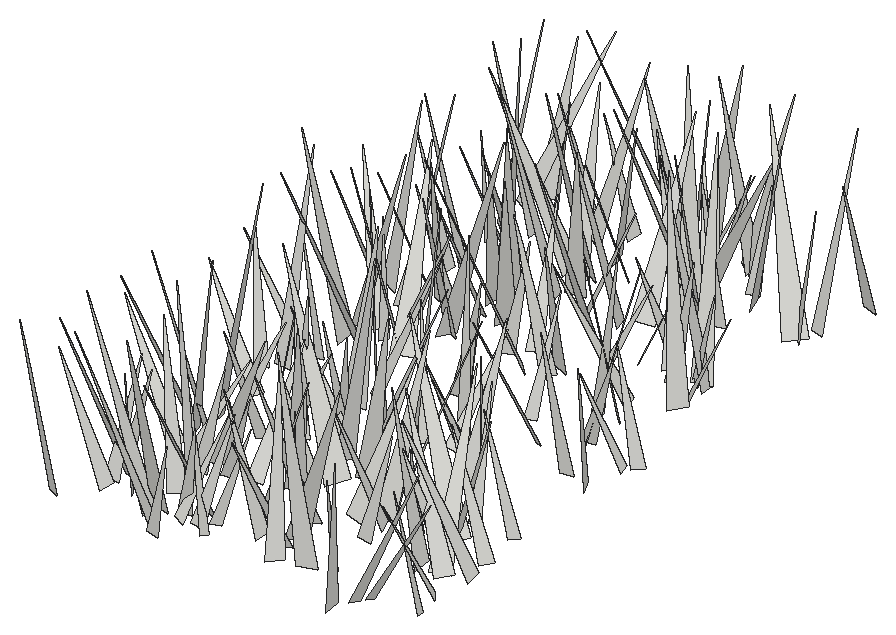
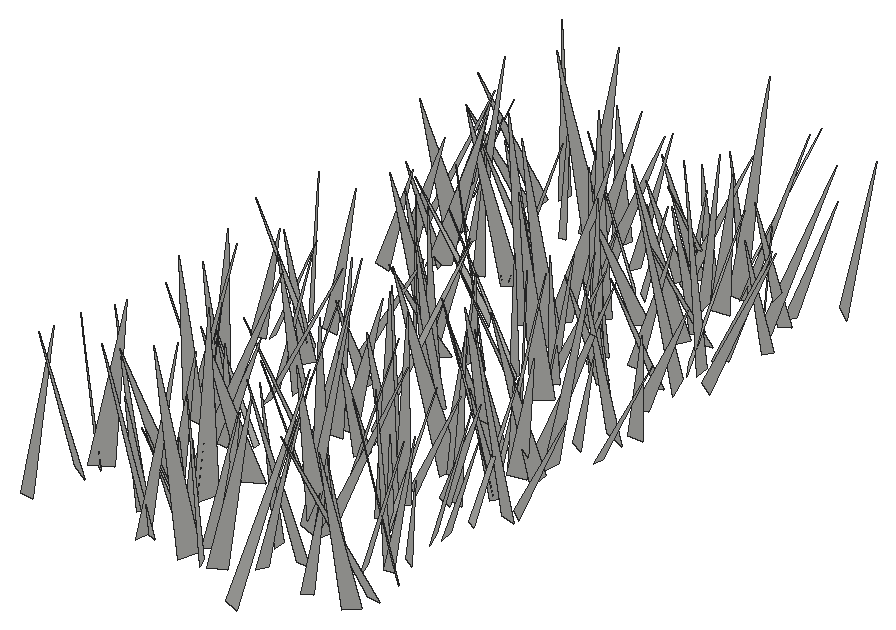
# SketchUp Ruby script. Lengths in inches.
U = 1.inch
M = Sketchup.active_model
def pt(a) = Geom::Point3d.new(a.map { |v| v * U })
def face(e, loops, mat)
  f = e.add_face(loops[0].map { |a| pt(a) })
  loops[1..].each { |l| e.add_face(l.map { |a| pt(a) }).erase! }
  f.material = f.back_material = mat if mat
  f
end
# faces: each face lists its corners as indices into pts; further lists are holes
def faces(e, pts, list, mat = nil) = list.each { |f| face(e, (f[0].is_a?(Array) ? f : [f]).map { |l| l.map { |i| pts[i] } }, mat) }
# xy, xz, yz: faces in a plane at the given z, y or x. An outline is a flat list of corners, or four numbers for a rectangle; further outlines are holes
def ring(l) = l.size == 4 ? [[l[0], l[1]], [l[2], l[1]], [l[2], l[3]], [l[0], l[3]]] : l.each_slice(2).to_a
def flat(e, list, mat, &to3) = list.each { |f| face(e, (f[0].is_a?(Array) ? f : [f]).map { |l| ring(l).map { |u, v| to3.(u, v) } }, mat) }
def xy(e, z, list, mat = nil) = flat(e, list, mat) { |x, y| [x, y, z] }
def xz(e, y, list, mat = nil) = flat(e, list, mat) { |x, z| [x, y, z] }
def yz(e, x, list, mat = nil) = flat(e, list, mat) { |y, z| [x, y, z] }
def lines(e, pts, list) = list.each { |a, b| e.add_line(pt(pts[a]), pt(pts[b])) }
# prism: a flat outline (further loops are holes) pulled along v
def prism(e, loops, v, mat = nil)
  f = face(e, loops, mat); d = Geom::Vector3d.new(v.map { |x| x * U })
  f.pushpull(f.normal.samedirection?(d) ? d.length : -d.length)
end
def box(e, o, s, mat = nil) = prism(e, [[o, [o[0] + s[0], o[1], o[2]], [o[0] + s[0], o[1] + s[1], o[2]], [o[0], o[1] + s[1], o[2]]]], [0, 0, s[2]], mat)
def at(x, y, z, deg = 0) = Geom::Transformation.translation(pt([x, y, z])) * Geom::Transformation.rotation(ORIGIN, Z_AXIS, deg.degrees)
def axes(o, x, y, z) = Geom::Transformation.new([*x, 0, *y, 0, *z, 0, *pt(o).to_a, 1])
def part(name) = M.definitions.add(name)
# library, detail: a bought-in or finely detailed component or shape, given as its bounding box
def library(name, o, s) = part(name).tap { |d| box(d.entities, o, s) }
def detail(e, o, s) = box(e.add_group.entities, o, s)
def put(e, d, t, mat = nil) = e.add_instance(d, t).tap { |i| i.material = mat if mat }
def group(e, t, mat = nil) = e.add_group.tap { |g| g.transformation = t; g.material = mat if mat }.entities
root = M.entities
c1 = part("fur_instance\#9")
p = [[0.8125,0,1.79],[0.67,-0.02,1.48],[0,-0.11,0],[0,0.11,0]]
faces(c1.entities,p,[[0,1,2,3]])
put(root,c1,axes([454.59,89.14,-21.66],[-2.53868,-3.44184,0.53172],[-3.38696,2.28677,-1.36858],[-0.81085,1.22404,4.05193]))
put(root,c1,axes([454.88,80.51,-21.66],[-4.32306,0.06447,0.02072],[0.06687,4.27292,0.65655],[0.01068,-0.65679,4.2734]))
put(root,c1,axes([454.72,56.08,-21.66],[-3.28868,-4.79968,1.75844],[-5.10998,3.14053,-0.98472],[0.13097,2.01112,5.73434]))
put(root,c1,axes([455.49,68.98,-21.66],[-2.53227,-4.93937,0.36335],[-4.86121,2.40071,-1.24381],[-0.94765,0.88376,5.4095]))
put(root,c1,axes([454.92,76.75,-21.66],[-0.91318,4.58049,0.90258],[4.61205,0.74242,0.89849],[-0.72428,-1.04754,4.5834]))
put(root,c1,axes([456.35,93.99,-21.66],[-4.63616,-0.58897,0.33378],[-0.62989,4.59941,-0.63319],[0.24806,0.67142,4.63033]))
put(root,c1,axes([456.92,65.64,-21.66],[-4.48303,2.72425,0.35571],[2.72908,4.33728,1.17718],[-0.3165,-1.18832,5.11208]))
put(root,c1,axes([456.77,94.78,-21.66],[-5.59376,-1.56322,0.76508],[-1.67452,5.53596,-0.93185],[0.47433,1.10847,5.73284]))
put(root,c1,axes([456.88,73.71,-21.66],[-3.88022,2.75048,0.41463],[2.75578,3.70465,1.21426],[-0.37781,-1.22622,4.59857]))
put(root,c1,axes([456.91,58.71,-21.66],[-4.89818,0.93846,0.55806],[1.01529,4.8584,0.74127],[0.40164,-0.83642,4.93188]))
put(root,c1,axes([456.1,98.09,-21.66],[1.10778,3.32388,1.25845],[3.28018,-1.46364,0.97838],[-1.36832,-0.8177,3.36424]))
put(root,c1,axes([457.63,100.73,-21.66],[-6.22819,-1.34042,0.61243],[-1.44458,6.07908,-1.38568],[0.29149,1.48668,6.21828]))
put(root,c1,axes([455.85,77.6875,-21.66],[1.84085,7.01016,1.12106],[6.97031,-2.00445,1.08846],[-1.34679,-0.79226,7.16563]))
put(root,c1,axes([454.67,89.88,-21.66],[2.76981,6.05425,2.08045],[6.39697,-2.70498,-0.64491],[-0.24704,-2.16406,6.62646]))
put(root,c1,axes([457.2,60.6875,-21.66],[-2.8111,-5.64649,0.53318],[-5.64839,2.7334,-0.83291],[-0.51273,0.84565,6.25232]))
put(root,c1,axes([456.08,91.8,-21.66],[-3.01664,-4.03882,0.35129],[-3.9528,3.02747,0.86334],[0.90049,-0.2406,4.96657]))
put(root,c1,axes([456.72,82.96,-21.66],[6.73753,-0.02978,4.19134],[0.53715,-7.86314,-0.91932],[-4.15689,-1.06433,6.67458]))
put(root,c1,axes([457.66,85.21,-21.66],[-2.82943,5.24506,0.49337],[5.22615,2.72388,1.01368],[-0.66438,-0.91081,5.87271]))
put(root,c1,axes([455.375,100.17,-21.66],[4.64173,5.41011,1.53464],[5.42173,-4.8336,0.64123],[-1.49305,-0.73288,7.09956]))
put(root,c1,axes([455.2,104.96,-21.66],[2.82826,-4.43632,2.67471],[-5.15951,-2.68482,1.00262],[-0.46309,2.81866,5.16476]))
put(root,c1,axes([457.86,67.78,-21.66],[-5.59539,-3.44886,0.89561],[-3.54081,5.56848,-0.67808],[0.39927,1.05,6.53783]))
put(root,c1,axes([457.12,79.87,-21.66],[0.68239,3.8164,1.4602],[3.78451,-1.14857,1.23331],[-1.54098,-1.13076,3.67553]))
put(root,c1,axes([457.93,82.92,-21.66],[-3.16334,-6.14078,0.476],[-6.132,3.08971,-0.89149],[-0.57823,0.82883,6.8499]))
put(root,c1,axes([455.2,63.04,-21.66],[1.8239,-3.22944,0.77362],[-3.28665,-1.6292,0.94764],[0.47508,1.1273,3.58579]))
put(root,c1,axes([456.39,99.71,-21.66],[-0.44013,-4.40012,0.04518],[-4.35564,0.44209,0.62427],[0.62566,-0.01764,4.37779]))
put(root,c1,axes([454.86,103.1,-21.66],[2.4491,6.4359,0.09226],[6.32974,-2.3903,-1.28384],[1.16776,-0.54137,6.7654]))
put(root,c1,axes([457.49,98.48,-21.66],[-6.13991,-1.94187,2.86824],[-2.65031,6.39227,-1.34568],[2.23013,2.25037,6.2975]))
put(root,c1,axes([456.54,59.68,-21.66],[1.07751,-3.9043,2.33703],[-4.53898,-0.75293,0.83488],[0.32078,2.46086,3.96327]))
put(root,c1,axes([456.25,84.875,-21.66],[6.19902,-0.22924,1.58295],[-0.50577,-6.29178,1.06951],[-1.51739,1.16065,6.11037]))
put(root,c1,axes([456.9,70,-21.66],[7.33246,2.99097,2.42144],[2.72494,-7.71469,1.27771],[-2.71735,0.33456,7.81527]))
put(root,c1,axes([456.49,76.91,-21.66],[3.46775,1.51161,0.84573],[1.722,-3.21287,-1.3182],[-0.18693,-1.55498,3.54578]))
put(root,c1,axes([456.85,88.32,-21.66],[2.18192,-3.03993,1.35648],[-3.32882,-1.9865,0.90262],[0.01238,1.6293,3.63142]))
put(root,c1,axes([458.72,58.99,-21.66],[-3.32365,-1.7064,1.24939],[-2.04417,3.18881,-1.08271],[0.54234,1.56176,3.57578]))
put(root,c1,axes([459.19,90.5625,-21.66],[-0.15517,3.72025,1.9318],[3.94772,-0.52047,1.31942],[-1.40985,-1.86683,3.48188]))
put(root,c1,axes([458.74,84.32,-21.66],[-3.88558,0.60859,0.85055],[0.43871,3.91906,-0.80001],[0.9494,0.67978,3.85072]))
put(root,c1,axes([456.9,67.54,-21.66],[6.76883,1.43904,1.95286],[1.74836,-6.90673,-0.9705],[-1.68159,-1.38844,6.85171]))
put(root,c1,axes([461.03,57.89,-21.66],[-7.48937,-0.81173,0.36322],[-0.84224,7.4632,-0.68756],[0.28542,0.72333,7.50179]))
put(root,c1,axes([457.81,87.38,-21.66],[5.71474,5.0925,1.62445],[5.00095,-5.93344,1.00766],[-1.88756,-0.30227,7.58791]))
put(root,c1,axes([459.09,85.15,-21.66],[-4.71687,-4.84842,1.35584],[-4.8132,4.8877,0.73342],[1.47602,0.44449,6.72444]))
put(root,c1,axes([459.44,95.77,-21.66],[-4.54245,-0.30979,1.16713],[-0.64985,4.4561,-1.34644],[1.01777,1.46262,4.34936]))
put(root,c1,axes([459.21,96.65,-21.66],[-3.58338,-3.97137,0.418],[-3.89573,3.60001,0.80641],[0.87736,-0.23507,5.28792]))
put(root,c1,axes([458.54,105.23,-21.66],[3.22144,-2.0672,0.86258],[-1.86043,-3.31076,-0.98626],[-1.24746,-0.40075,3.69841]))
put(root,c1,axes([458.46,90.32,-21.66],[-1.39495,-5.41554,1.57218],[-5.52882,1.63221,0.71678],[1.10996,1.3242,5.54619]))
put(root,c1,axes([459.18,100.59,-21.66],[-4.14484,-0.82966,2.07391],[-1.4546,4.32013,-1.17886],[1.69516,1.67847,4.05935]))
put(root,c1,axes([457.67,70.83,-21.66],[1.33461,3.80482,0.72121],[3.71713,-1.04467,-1.36733],[1.08616,-1.09999,3.79319]))
put(root,c1,axes([462.34,56.64,-21.66],[-6.31151,-2.93767,0.11387],[-2.9284,6.25835,-0.85765],[-0.25951,0.82534,6.90866]))
put(root,c1,axes([462.375,98.66,-21.66],[-7.38136,0.22251,0.33251],[0.26326,7.32737,0.9407],[0.30128,-0.95116,7.32455]))
put(root,c1,axes([460.87,60.8,-21.66],[-1.86081,5.49202,1.44787],[5.66351,1.67938,0.90859],[-0.42807,-1.65488,5.72707]))
put(root,c1,axes([460.64,69.7,-21.66],[0.6809,-4.24063,0.83858],[-4.19337,-0.85411,-0.91428],[-1.04966,0.66131,4.19651]))
put(root,c1,axes([461.59,90.7,-21.66],[-2.18116,-3.44946,0.52539],[-3.41914,1.9894,-1.13316],[-0.6959,1.0372,3.92074]))
put(root,c1,axes([460.92,83.4375,-21.66],[-3.48559,6.14429,0.41822],[6.11379,3.5101,-0.61419],[0.74073,-0.05879,7.03735]))
put(root,c1,axes([461.92,61.15,-21.66],[-6.95078,-0.2098,1.40903],[-0.48679,6.94525,-1.36721],[1.33881,1.43604,6.81821]))
put(root,c1,axes([458.67,64.59,-21.66],[1.67584,3.97009,0.12724],[3.80521,-1.56498,-1.28741],[1.13936,-0.61275,4.1125]))
put(root,c1,axes([461.38,109.32,-21.66],[-3.81436,-7.20009,0.2192],[-7.12697,3.80817,1.069],[1.0467,-0.30859,8.07762]))
put(root,c1,axes([461.8125,79.7,-21.66],[3.98122,4.30027,2.75674],[4.211,-4.74141,1.31475],[-2.89126,-0.98426,5.71085]))
put(root,c1,axes([460.34,63.76,-21.66],[2.46707,-3.42013,1.11602],[-3.59628,-2.30764,0.87798],[0.09798,1.4166,4.12467]))
put(root,c1,axes([461.14,58.67,-21.66],[-1.28259,-7.19659,1.19017],[-7.23451,1.40948,0.72639],[0.93233,1.03678,7.27381]))
put(root,c1,axes([463.77,95.43,-21.66],[-6.93543,-2.32629,0.88421],[-2.41004,6.93097,-0.66862],[0.62063,0.91853,7.28456]))
put(root,c1,axes([461.41,87.61,-21.66],[-1.87294,-5.65903,1.00828],[-5.62978,2.02003,0.87988],[1.16052,0.66634,5.89562]))
put(root,c1,axes([462.74,71.13,-21.66],[-1.18349,4.29439,0.91251],[4.36217,1.04349,0.74676],[-0.49586,-1.06979,4.39144]))
put(root,c1,axes([459.84,84.73,-21.66],[4.56637,-2.19972,0.30987],[-2.21681,-4.46657,0.96025],[0.14341,0.99877,4.97679]))
put(root,c1,axes([461.03,92.55,-21.66],[5.82388,-2.11588,0.96568],[-1.89422,-5.82584,-1.34106],[-1.34958,-0.95373,6.04946]))
put(root,c1,axes([460.71,94.49,-21.66],[2.24537,-6.9608,0.71668],[-6.96969,-2.1575,0.8813],[0.62434,0.94895,7.26069]))
put(root,c1,axes([462.875,104.38,-21.66],[-4.43499,0.78648,1.49873],[1.10021,4.53377,0.87655],[1.28619,-1.16631,4.41807]))
put(root,c1,axes([464.1,73.45,-21.66],[-4.45422,0.97791,0.2811],[1.01486,4.3608,0.91044],[0.07343,-0.95002,4.4685]))
put(root,c1,axes([461.14,102.37,-21.66],[2.20928,6.37096,1.50715],[6.50914,-1.9672,-1.22586],[0.70121,-1.81177,6.63078]))
put(root,c1,axes([461.02,72.41,-21.66],[2.09245,-2.98815,0.44058],[-2.87886,-1.81085,1.39087],[0.91397,1.13723,3.37237]))
put(root,c1,axes([460.37,65.39,-21.66],[4.49175,-3.99144,0.42922],[-3.97143,-4.32409,1.3497],[0.58618,1.28931,5.8554]))
put(root,c1,axes([464.54,59.9,-21.66],[-2.68226,-4.58353,0.12394],[-4.53778,2.63294,-0.83358],[-0.65781,0.52677,5.24485]))
put(root,c1,axes([462.06,71.75,-21.66],[-0.22733,-5.68785,1.31588],[-5.73337,0.46581,1.02292],[1.10075,1.2515,5.59972]))
put(root,c1,axes([461.41,87.27,-21.66],[7.18053,-1.42617,1.70446],[-1.71997,-7.21687,1.20732],[-1.40743,1.54336,7.22055]))
put(root,c1,axes([463.36,97.97,-21.66],[-4.06355,5.05875,1.67662],[5.05755,4.32523,-0.79246],[1.68023,-0.78477,6.44014]))
put(root,c1,axes([463.72,98.79,-21.66],[-3.21608,-6.87634,1.40534],[-6.91778,3.36666,0.64196],[1.18463,0.99184,7.56406]))
put(root,c1,axes([462.02,64.46,-21.66],[2.06201,-3.51619,0.27094],[-3.44771,-1.94389,1.0117],[0.74186,0.73932,3.94867]))
put(root,c1,axes([463.72,74.08,-21.66],[-3.9744,-0.24759,1.6573],[0.13335,4.20562,0.94807],[1.67038,-0.92483,3.8676]))
put(root,c1,axes([462.55,76.48,-21.66],[2.84119,-6.18581,2.36185],[-6.62137,-2.65127,1.02137],[0.00779,2.57322,6.73004]))
put(root,c1,axes([462.91,55.77,-21.66],[0.44262,-3.83329,1.02735],[-3.85493,-0.16968,1.02773],[0.94293,1.1057,3.71938]))
put(root,c1,axes([462.92,59.09,-21.66],[1.90373,-3.64825,0.45227],[-3.65968,-1.83258,0.622],[0.34793,0.68584,4.0678]))
put(root,c1,axes([465.58,57.68,-21.66],[-4.50739,-0.00087,0.31518],[-0.09503,4.31184,-1.34718],[0.30051,1.35052,4.30136]))
put(root,c1,axes([463.1,58.17,-21.66],[1.23248,3.89294,0.26564],[3.83774,-1.15903,-0.82034],[0.70519,-0.49622,4.00013]))
put(root,c1,axes([463.73,65.06,-21.66],[-1.59492,4.69203,0.53683],[4.53057,1.68008,-1.22409],[1.33316,-0.09626,4.80214]))
put(root,c1,axes([463.3,69.8,-21.66],[0.07384,-6.03784,2.03973],[-6.28438,0.27016,1.02718],[1.05955,2.02311,5.95028]))
put(root,c1,axes([463.31,74.45,-21.66],[0.57309,-4.07864,0.58369],[-4.03575,-0.43699,0.90892],[0.82985,0.69149,4.01716]))
put(root,c1,axes([463.23,90.91,-21.66],[5.78336,-2.78291,1.02515],[-2.6557,-5.85961,-0.92463],[-1.32013,-0.40388,6.35113]))
put(root,c1,axes([465.04,106.18,-21.66],[3.86572,-4.28586,2.24353],[-4.19582,-4.39988,-1.17556],[-2.40771,0.7863,5.6507]))
put(root,c1,axes([463.03,77.99,-21.66],[3.15484,4.86518,0.39731],[4.85003,-3.07066,-0.91053],[0.55227,-0.82578,5.72659]))
put(root,c1,axes([465.85,62.36,-21.66],[-2.1087,-2.96786,0.97974],[-3.12443,1.97245,-0.74971],[-0.07759,1.23123,3.56269]))
put(root,c1,axes([463.83,101.45,-21.66],[5.32416,0.8497,1.29821],[1.01973,-5.41351,-0.63884],[-1.1694,-0.85204,5.35356]))
put(root,c1,axes([467.91,68.21,-21.66],[-7.19785,3.45896,0.52945],[3.49375,7.17168,0.64382],[0.19618,-0.81015,7.95983]))
put(root,c1,axes([466.17,67.86,-21.66],[-3.68845,0.83243,0.84341],[0.99836,3.66829,0.74556],[0.6384,-0.92717,3.70698]))
put(root,c1,axes([467.9375,86.83,-21.66],[-5.60021,-5.8066,0.30959],[-5.79691,5.54128,-0.92996],[-0.45638,0.8674,8.01337]))
put(root,c1,axes([465.66,100.15,-21.66],[-3.10311,-4.08719,0.56583],[-3.96021,3.14894,1.02739],[1.15846,-0.18348,5.02781]))
put(root,c1,axes([464.53,96.34,-21.66],[2.07468,-5.92746,1.15005],[-6.03286,-1.98482,0.6533],[0.24901,1.299,6.24598]))
put(root,c1,axes([464.5,58.31,-21.66],[-0.11814,4.24138,1.60816],[4.31681,0.59918,-1.26317],[1.39308,-1.49704,4.05064]))
put(root,c1,axes([465.31,59.2,-21.66],[3.08965,-1.86478,1.07968],[-2.12915,-2.93231,1.02827],[-0.33144,1.45368,3.45919]))
put(root,c1,axes([467.08,89.04,-21.66],[-3.56448,3.67904,0.44666],[3.56023,3.5714,-1.00507],[1.02934,0.38746,5.02301]))
put(root,c1,axes([465.8,75.32,-21.66],[3.91592,-0.46866,0.80636],[-0.26131,-3.89224,-0.99321],[-0.89531,-0.91384,3.81675]))
put(root,c1,axes([469.09,95.16,-21.66],[-7.24522,-3.15461,1.03201],[-3.28219,7.17812,-1.10079],[0.49381,1.42581,7.82516]))
put(root,c1,axes([465.88,87.78,-21.66],[2.99214,-2.75371,1.44433],[-3.06357,-2.95389,0.71483],[-0.53251,1.52102,4.0031]))
put(root,c1,axes([468.21,101.79,-21.66],[-1.43576,4.62376,1.24523],[4.74317,1.1948,1.0324],[-0.65727,-1.47798,4.73019]))
put(root,c1,axes([467.14,104.4,-21.66],[-3.93498,0.71077,2.15609],[1.47172,4.08376,1.33974],[1.72857,-1.85895,3.76754]))
put(root,c1,axes([466.21,106.26,-21.66],[-4.16703,-2.76107,2.92288],[-2.78486,5.0182,0.77013],[2.90022,0.85149,4.93909]))
put(root,c1,axes([466.09,66.28,-21.66],[6.0824,-3.06076,1.36011],[-2.97573,-6.23245,-0.71791],[-1.53726,-0.04598,6.77115]))
put(root,c1,axes([466.49,70.67,-21.66],[7.07212,-1.1156,2.41076],[-1.38462,-7.39913,0.63784],[-2.26697,1.03896,7.1311]))
put(root,c1,axes([468.52,59.85,-21.66],[-5.18821,0.426,1.12668],[0.56814,5.25845,0.62796],[1.06213,-0.73187,5.16766]))
put(root,c1,axes([467.98,93.45,-21.66],[-2.86218,-6.85746,0.77217],[-6.83354,2.93291,0.71683],[0.96112,0.43167,7.39614]))
put(root,c1,axes([466.57,82.47,-21.66],[1.64053,-3.56149,0.70323],[-3.59089,-1.47867,0.88831],[0.53314,0.99969,3.81922]))
put(root,c1,axes([469.07,75.58,-21.66],[-4.35702,1.54483,0.37411],[1.45493,4.3157,-0.87633],[0.64002,0.7059,4.53896]))
put(root,c1,axes([465.8,75.08,-21.66],[4.98455,3.49636,0.32674],[3.50629,-4.92427,-0.79656],[0.19289,-0.83908,6.03621]))
put(root,c1,axes([469.59,87.31,-21.66],[0.51311,-4.91857,2.52241],[-5.22585,-1.25725,-1.38854],[-1.80151,2.24614,4.74633]))
put(root,c1,axes([466.5,95.05,-21.66],[3.8277,2.64651,0.3376],[2.6435,-3.68235,-1.10521],[0.36045,-1.09797,4.52038]))
put(root,c1,axes([468.48,75.08,-21.66],[5.2038,5.70361,2.35891],[5.67233,-5.63566,1.11317],[-2.43315,-0.93989,7.64013]))
put(root,c1,axes([466.72,62.06,-21.66],[4.42426,3.38365,0.88099],[3.49585,-4.30744,-1.01209],[-0.06566,-1.34021,5.47712]))
put(root,c1,axes([466.98,81.61,-21.66],[2.1882,-4.93746,0.79161],[-4.93819,-1.99768,1.19031],[0.78701,1.19336,5.26781]))
put(root,c1,axes([469.26,62.12,-21.66],[2.90611,1.79436,1.69144],[1.585,-3.36196,0.84331],[-1.88904,-0.06039,3.30969]))
put(root,c1,axes([467.42,106.01,-21.66],[6.54433,-2.87567,1.841],[-3.10892,-6.66403,0.64215],[-1.41189,1.3447,7.11937]))
put(root,c1,axes([469.91,63.2,-21.66],[0.31088,-6.10314,0.84199],[-6.04835,-0.46277,-1.12122],[-1.17245,0.76905,6.00731]))
put(root,c1,axes([470.23,102.375,-21.66],[-1.23415,4.06964,0.18802],[4.01431,1.18128,0.78126],[-0.69473,-0.40381,4.18028]))
put(root,c1,axes([470.07,103.36,-21.66],[-3.57041,1.71359,0.7726],[1.61509,3.64514,-0.62093],[0.96166,0.24019,3.91135]))
put(root,c1,axes([470.6,59.71,-21.66],[-0.13118,-4.53208,0.33432],[-4.41868,0.04908,-1.06843],[-1.06148,0.35576,4.40629]))
put(root,c1,axes([470.54,77.57,-21.66],[1.55743,6.34801,1.89562],[6.44853,-1.89902,1.06134],[-1.51893,-1.55328,6.44953]))
put(root,c1,axes([471.06,57.91,-21.66],[-5.70691,2.72816,1.15825],[2.57005,5.80682,-1.01437],[1.47624,0.43731,6.24361]))
put(root,c1,axes([471.09,99.68,-21.66],[-7.16118,3.19135,1.99245],[3.1192,7.43157,-0.69239],[2.1036,-0.15533,7.80947]))
put(root,c1,axes([468.65,104.25,-21.66],[3.29309,2.39527,0.08068],[2.3726,-3.23886,-0.68467],[0.3385,-0.60058,4.0141]))
put(root,c1,axes([470.13,96.13,-21.66],[-2.04424,6.85145,0.72305],[6.79433,2.1298,-0.97223],[1.1412,-0.40704,7.08351]))
put(root,c1,axes([471.23,105.86,-21.66],[-6.84332,-0.22544,2.15666],[-0.013,7.14388,0.70553],[2.16837,-0.66867,6.81058]))
put(root,c1,axes([469.74,88.3,-21.66],[-1.23587,-5.65616,0.92472],[-5.5483,1.41785,1.25724],[1.43652,0.61007,5.65145]))
put(root,c1,axes([469.2,69.57,-21.66],[2.15737,-6.51602,1.69287],[-6.69271,-1.88316,1.28061],[0.7294,1.99342,6.74336]))
put(root,c1,axes([473.25,98.28,-21.66],[-4.28269,-7.03673,0.88853],[-7.06243,4.13524,-1.29164],[-0.65353,1.42504,8.13564]))
put(root,c1,axes([470.28,103.18,-21.66],[3.75823,0.40452,0.85087],[0.18545,-3.74836,0.96295],[-0.9237,0.89332,3.65522]))
put(root,c1,axes([471.98,75.99,-21.66],[0.37183,-3.94608,0.38846],[-3.8933,-0.43727,-0.71534],[-0.75144,0.31297,3.89847]))
put(root,c1,axes([470.79,75.97,-21.66],[-0.63847,4.33122,0.11328],[4.14955,0.64421,-1.24344],[1.2464,0.07394,4.19773]))
put(root,c1,axes([472.22,76.02,-21.66],[-3.37943,-0.96857,0.84627],[-0.6019,3.29348,1.36586],[1.13667,-1.13567,3.23931]))
put(root,c1,axes([473.23,58.45,-21.66],[0.00148,-6.83986,3.17541],[-7.42007,-0.56775,-1.21947],[-1.34516,3.12424,6.73027]))
put(root,c1,axes([472.18,99.15,-21.66],[4.90048,2.76624,3.25214],[3.64641,-5.28694,-0.99757],[-2.22086,-2.5767,5.5382]))
put(root,c1,axes([472.29,82.08,-21.66],[-3.28423,2.60896,0.74342],[2.31234,3.30268,-1.37511],[1.4186,0.65664,3.96257]))
put(root,c1,axes([470.91,105.56,-21.66],[3.79421,5.57197,1.64798],[5.81056,-3.63804,-1.07735],[0.00109,-1.96889,6.65448]))
put(root,c1,axes([474.71,79.95,-21.66],[-2.69174,-3.80387,0.07847],[-3.66679,2.56798,-1.29661],[-1.01502,0.8106,4.47591]))
put(root,c1,axes([470.29,102.64,-21.66],[5.56558,-2.4926,0.3103],[-2.49513,-5.39934,1.38077],[0.28926,1.38533,5.93988]))
put(root,c1,axes([470.39,60.97,-21.66],[5.68552,-4.38043,0.51347],[-4.40819,-5.61738,0.88871],[0.14016,1.01677,7.12204]))
put(root,c1,axes([473.71,65.68,-21.66],[-4.5248,-1.88356,0.71077],[-1.69814,4.51006,1.14127],[1.08134,-0.799,4.76646]))
put(root,c1,axes([471.68,65.15,-21.66],[0.68062,5.93772,0.86921],[5.89172,-0.495,-1.23203],[1.14003,-0.98679,5.84823]))
put(root,c1,axes([471.55,70.58,-21.66],[5.03516,3.5658,0.22039],[3.50469,-5.00395,0.89105],[-0.69327,0.6016,6.10523]))
put(root,c1,axes([474.1875,98.76,-21.66],[-0.90978,-4.59674,2.27002],[-5.08569,0.51819,-0.98893],[-0.64715,2.39002,4.58036]))
put(root,c1,axes([473.26,103.3,-21.66],[-1.45732,3.49071,1.72371],[3.67662,1.83923,-0.61623],[1.28012,-1.30851,3.73217]))
put(root,c1,axes([474.83,93.6,-21.66],[0.84597,-3.78981,1.14812],[-3.67965,-1.18614,-1.20406],[-1.46323,0.79177,3.69169]))
put(root,c1,axes([475.91,87.58,-21.66],[-5.4104,-1.19331,0.05848],[-1.15989,5.3113,1.06983],[0.28647,-1.03242,5.43616]))
put(root,c1,axes([472.39,89.05,-21.66],[2.24479,3.42751,0.35228],[3.3467,-2.06895,-1.19586],[0.81948,-0.93948,3.91878]))
put(root,c1,axes([473.25,66.32,-21.66],[-1.23701,6.48468,1.94316],[6.59867,1.59608,-1.12573],[1.51147,-1.6609,6.50492]))
put(root,c1,axes([475.11,92.4375,-21.66],[-3.68366,1.92684,0.76086],[1.83141,3.75443,-0.64122],[0.96827,0.22919,4.10742]))
put(root,c1,axes([474.17,74.86,-21.66],[-3.42009,-2.62307,1.97794],[-2.56254,3.91671,0.76324],[2.05575,0.51835,4.24205]))
put(root,c1,axes([472.9375,92.37,-21.66],[3.88446,1.51086,0.00017],[1.46105,-3.75628,-1.06181],[0.38475,-0.98965,4.03042]))
put(root,c1,axes([473.83,63.45,-21.66],[1.31447,-3.85278,1.5031],[-4.0825,-0.95693,1.11736],[0.66058,1.75255,3.91449]))
put(root,c1,axes([474.28,73.29,-21.66],[-2.07384,5.25709,1.74566],[5.26815,2.4479,-1.11335],[1.712,-1.16445,5.54061]))
put(root,c1,axes([475.28,85.11,-21.66],[5.18015,0.30458,2.40247],[-0.20645,-5.59667,1.15468],[-2.41288,1.13276,5.059]))
put(root,c1,axes([474.52,59.61,-21.66],[-1.23844,-4.00226,0.78585],[-3.84524,1.41955,1.16979],[1.36007,0.36904,4.02286]))
put(root,c1,axes([476.78,85.4,-21.66],[-4.01127,-3.66818,1.32519],[-3.89401,3.87381,-1.06408],[0.2199,1.68524,5.33044]))
put(root,c1,axes([474.31,65.83,-21.66],[3.53808,2.09554,0.91862],[2.27584,-3.39762,-1.01485],[-0.23603,-1.34836,3.98489]))
put(root,c1,axes([474.12,102.32,-21.66],[6.26752,1.77798,1.53658],[2.00319,-6.33057,-0.84565],[-1.22862,-1.25168,6.45971]))
put(root,c1,axes([478.47,67.07,-21.66],[-6.09178,4.42452,0.24879],[4.41982,6.03543,0.88707],[-0.32169,-0.86331,7.47659]))
put(root,c1,axes([478.58,92.04,-21.66],[-7.60093,-1.69118,1.08047],[-1.85126,7.54274,-1.21718],[0.77483,1.43129,7.69108]))
put(root,c1,axes([475.7,66.55,-21.66],[0.30074,-4.21199,0.28121],[-4.14735,-0.24225,0.80695],[0.78703,0.33293,4.14489]))
put(root,c1,axes([477.91,92.35,-21.66],[-0.32528,8.12923,0.88129],[8.06717,0.17507,1.36272],[-1.33486,-0.92294,8.0208]))
put(root,c1,axes([478.98,100.44,-21.66],[-5.24663,5.623,0.95369],[5.70188,5.20042,0.70642],[0.12741,-1.17997,7.65808]))
put(root,c1,axes([478.7,88.97,-21.66],[-7.32985,2.37013,1.25415],[2.21242,7.40801,-1.06942],[1.51512,0.64882,7.62892]))
put(root,c1,axes([477.98,69.39,-21.66],[0.35019,4.61175,0.40741],[4.56098,-0.41379,0.76359],[-0.79477,-0.34263,4.56155]))
put(root,c1,axes([476.6,91.02,-21.66],[0.64184,-5.02818,1.67754],[-5.1921,-0.25617,1.21871],[1.0672,1.77778,4.9203]))
put(root,c1,axes([478.51,78,-21.66],[-0.10037,-5.00985,1.67679],[-5.24561,-0.10471,-0.62683],[-0.62754,1.67652,4.9715]))
put(root,c1,axes([478.71,63.16,-21.66],[-6.33484,-0.15602,2.15214],[0.09289,6.64883,0.75543],[2.15578,-0.74496,6.29157]))
put(root,c1,axes([477.64,55.42,-21.66],[5.74214,0.07937,1.80023],[0.34922,-5.94743,-0.85168],[-1.76782,-0.91707,5.67918]))
put(root,c1,axes([477.66,80.66,-21.66],[5.27233,3.79468,0.9806],[3.62511,-5.34626,1.19781],[-1.48988,0.42019,6.38454]))
put(root,c1,axes([477.5,92.22,-21.66],[2.1321,2.91958,1.28602],[3.18698,-1.87905,-1.01782],[0.14466,-1.63367,3.46899]))
put(root,c1,axes([480.66,62.98,-21.66],[-3.78677,4.88862,0.77178],[4.90876,3.58599,1.37062],[-0.63111,-1.44081,6.0299]))
put(root,c1,axes([477.02,82.01,-21.66],[2.31724,-3.70248,0.25487],[-3.62607,-2.19471,1.08527],[0.79054,0.78602,4.23086]))
put(root,c1,axes([479.73,64.29,-21.66],[-4.18916,1.41328,1.44955],[1.84035,4.04661,1.3732],[0.84361,-1.80976,4.20247]))
put(root,c1,axes([478.39,66.89,-21.66],[4.03699,1.00135,1.00845],[0.75439,-4.0837,1.03503],[-1.2044,0.79854,4.02849]))
put(root,c1,axes([479.47,101.99,-21.66],[2.76869,6.15296,0.77217],[6.00563,-2.8712,1.34513],[-1.54517,-0.13446,6.61174]))
put(root,c1,axes([480.25,63.1,-21.66],[-4.33285,5.33033,0.39838],[5.19442,4.31986,-1.30443],[1.26061,0.52067,6.74422]))
put(root,c1,axes([481.14,69.45,-21.66],[-1.35537,3.98703,1.26023],[4.07237,0.95801,1.34893],[-0.94888,-1.58348,3.98921]))
put(root,c1,axes([480.9,80.74,-21.66],[-3.67924,-0.76157,0.35539],[-0.68587,3.64327,0.70657],[0.48566,-0.62424,3.6902]))
put(root,c1,axes([478.91,100.68,-21.66],[3.62429,3.41254,1.71474],[3.78655,-3.51895,-1.00013],[-0.49783,-1.92166,4.87654]))
put(root,c1,axes([478.27,56.9375,-21.66],[5.14686,-0.10254,0.48257],[-0.21946,-5.00543,1.27711],[-0.44184,1.29176,4.98695]))
put(root,c1,axes([482.23,63.98,-21.66],[-5.87087,-0.65311,0.1721],[-0.62527,5.82501,0.77566],[0.25536,-0.75237,5.85594]))
put(root,c1,axes([481.77,65.87,-21.66],[-2.38269,3.95567,1.05235],[4.03891,2.07425,1.34786],[-0.66484,-1.57548,4.41677]))
put(root,c1,axes([478.4,90.43,-21.66],[3.77978,1.93812,0.15141],[1.88384,-3.56988,-1.33157],[0.48001,-1.25124,4.0336]))
put(root,c1,axes([480.22,106.37,-21.66],[-0.97227,-5.54065,0.71566],[-5.53732,1.05209,0.62249],[0.741,0.5921,5.59077]))
put(root,c1,axes([478.875,57.8,-21.66],[4.0967,-0.1052,0.02727],[-0.10864,-3.93802,1.12914],[0.00278,1.12946,3.93942]))
put(root,c1,axes([481.6,81.31,-21.66],[1.42744,-3.53628,2.17287],[-3.81125,-2.02664,-0.79456],[-1.64348,1.62839,3.72982]))
put(root,c1,axes([480.47,77.48,-21.66],[4.23333,1.58778,2.03705],[2.11026,-4.38143,-0.97034],[-1.48911,-1.69519,4.41595]))
put(root,c1,axes([482.51,58.24,-21.66],[-3.84784,-1.19504,0.32807],[-1.23606,3.62421,-1.29571],[-0.08892,1.33363,3.81512]))
put(root,c1,axes([481.8,60.63,-21.66],[-3.17916,-2.57933,0.00353],[-2.53731,3.12837,0.73174],[0.46373,-0.56605,4.02798]))
